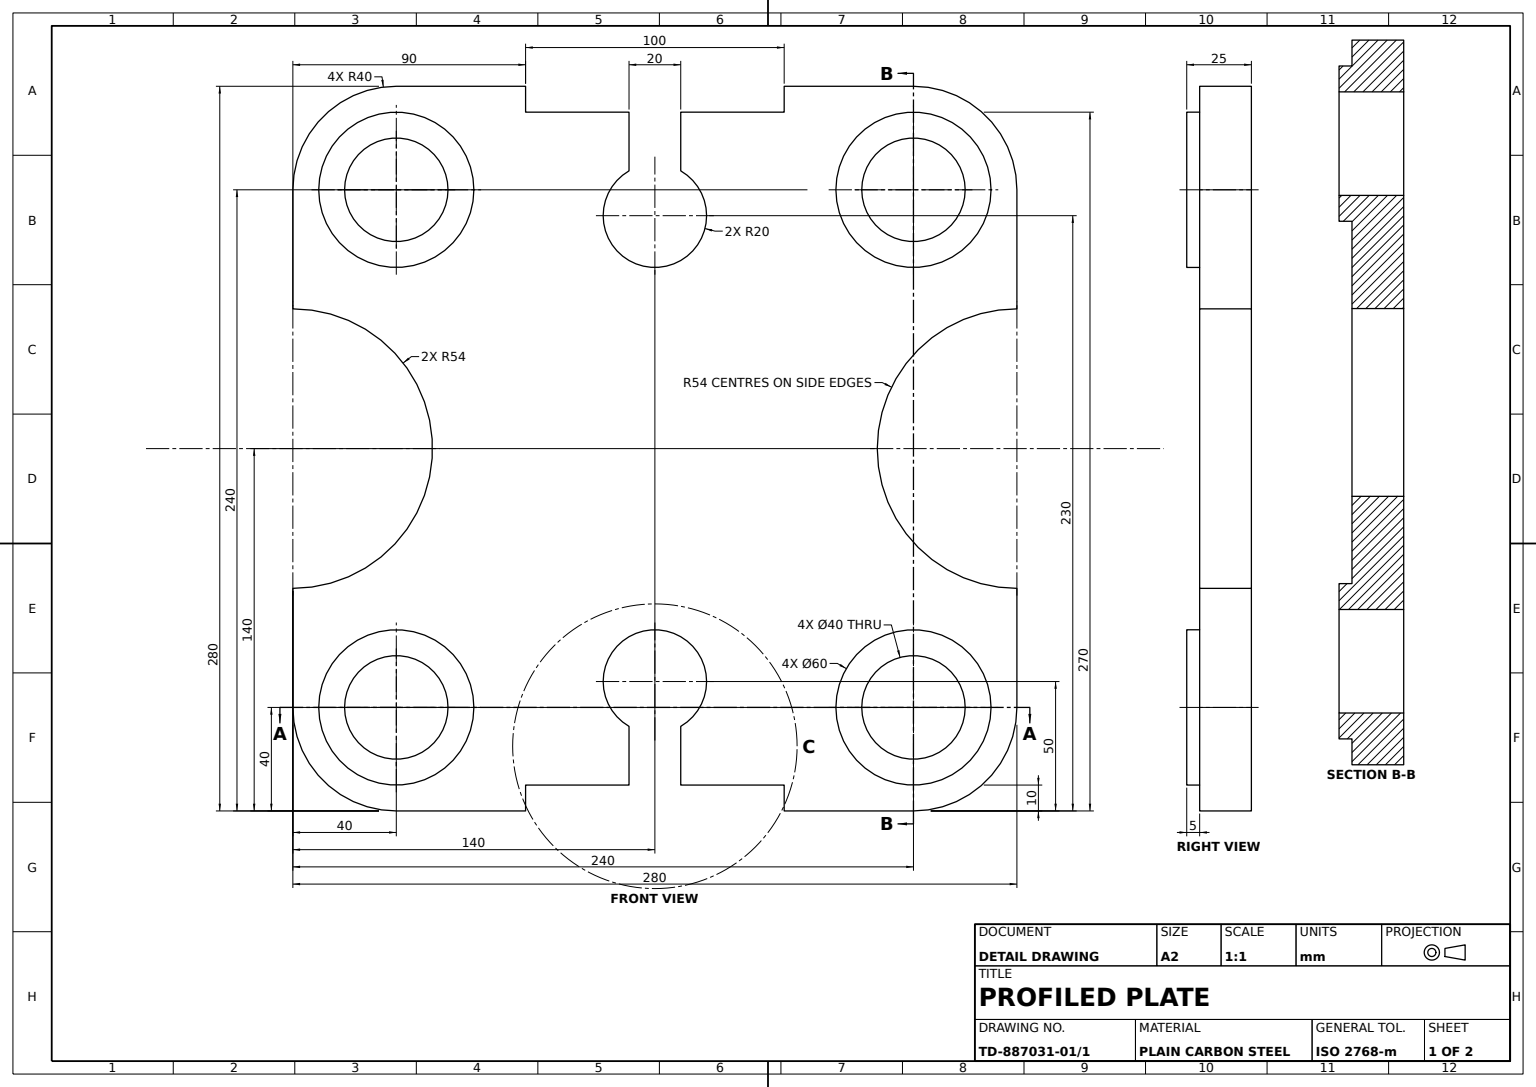
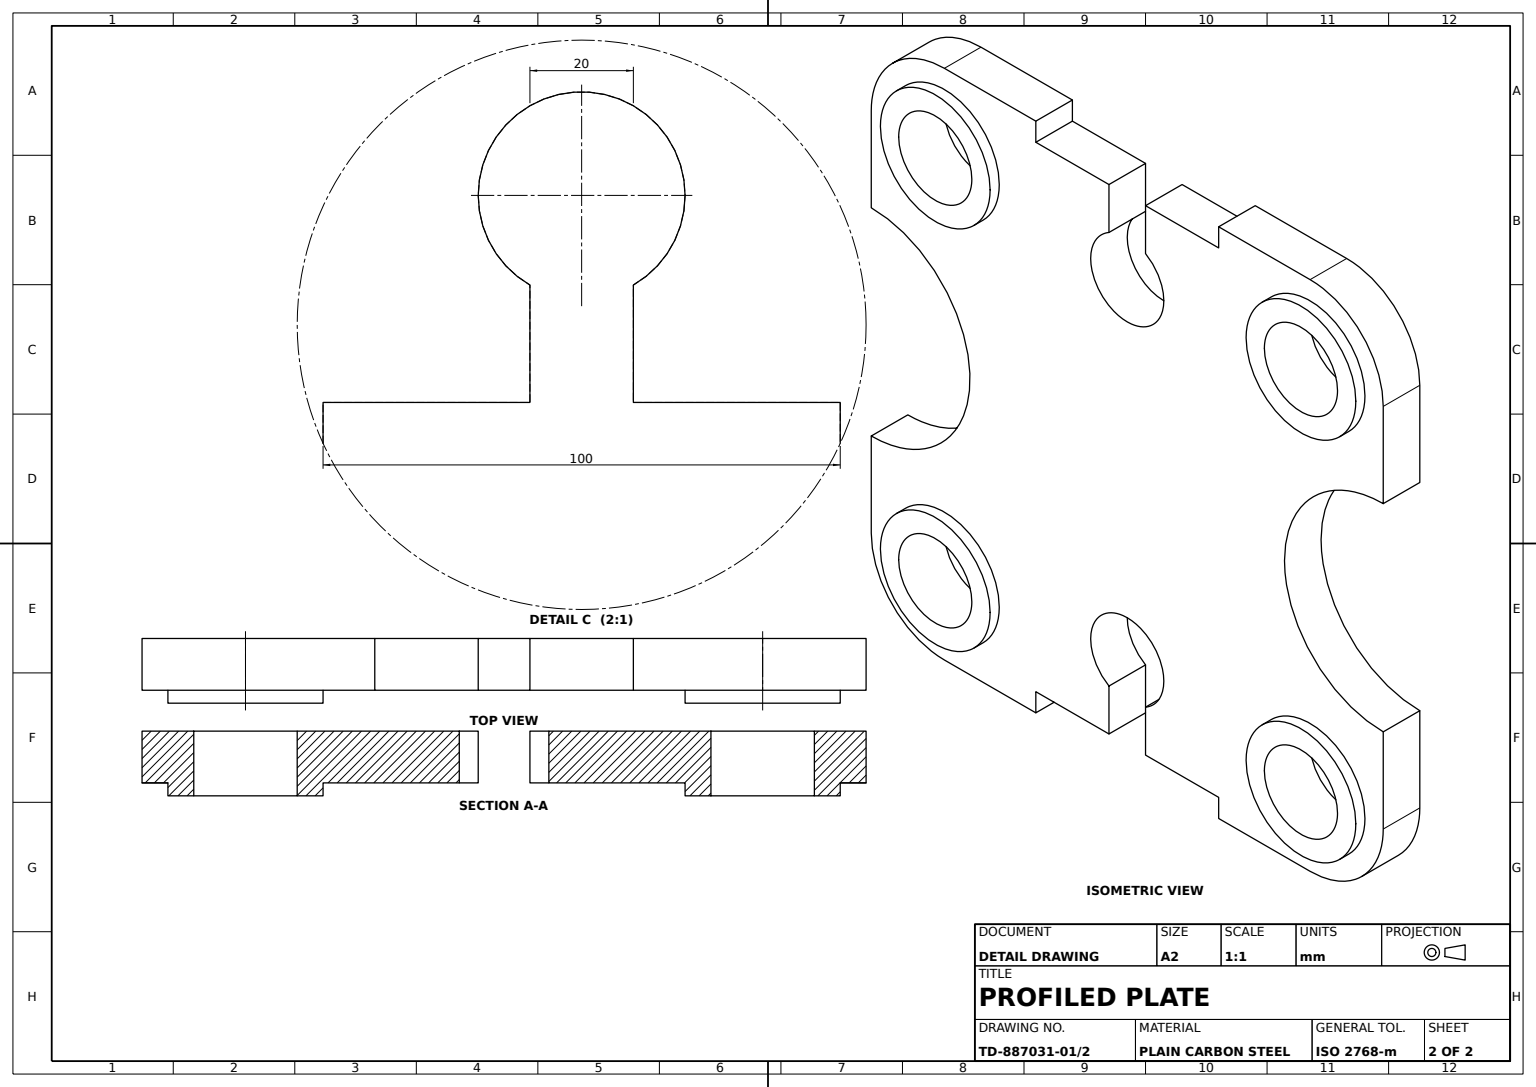
ISO-10303-21;
HEADER;
FILE_DESCRIPTION((''),'2;1');
FILE_NAME('','',(''),(''),'','','');
FILE_SCHEMA(('AUTOMOTIVE_DESIGN'));
ENDSEC;
DATA;
#1=APPLICATION_CONTEXT('');
#2=PRODUCT_CONTEXT('',#1,'mechanical');
#3=PRODUCT('','','',(#2));
#4=PRODUCT_DEFINITION_FORMATION('','',#3);
#5=PRODUCT_DEFINITION_CONTEXT('',#1,'design');
#6=PRODUCT_DEFINITION('','',#4,#5);
#7=PRODUCT_DEFINITION_SHAPE('','',#6);
#8=(LENGTH_UNIT()NAMED_UNIT(*)SI_UNIT(.MILLI.,.METRE.));
#9=(NAMED_UNIT(*)PLANE_ANGLE_UNIT()SI_UNIT($,.RADIAN.));
#10=(NAMED_UNIT(*)SI_UNIT($,.STERADIAN.)SOLID_ANGLE_UNIT());
#11=UNCERTAINTY_MEASURE_WITH_UNIT(LENGTH_MEASURE(1.E-05),#8,'distance_accuracy_value','');
#12=(GEOMETRIC_REPRESENTATION_CONTEXT(3)GLOBAL_UNCERTAINTY_ASSIGNED_CONTEXT((#11))GLOBAL_UNIT_ASSIGNED_CONTEXT((#8,#9,#10))REPRESENTATION_CONTEXT('',''));
#13=CARTESIAN_POINT('',(120.,230.,20.));
#14=VERTEX_POINT('',#13);
#15=CARTESIAN_POINT('',(120.,230.,0.));
#16=VERTEX_POINT('',#15);
#17=DIRECTION('',(0.,0.,-1.));
#18=VECTOR('',#17,1000.);
#19=LINE('',#13,#18);
#20=EDGE_CURVE('',#14,#16,#19,.T.);
#21=ORIENTED_EDGE('',*,*,#20,.T.);
#22=CARTESIAN_POINT('',(130.,247.320508,0.));
#23=VERTEX_POINT('',#22);
#24=CARTESIAN_POINT('',(140.,230.,0.));
#25=DIRECTION('',(1.,0.,0.));
#26=AXIS2_PLACEMENT_3D('',#24,#17,#25);
#27=CIRCLE('',#26,20.);
#28=EDGE_CURVE('',#16,#23,#27,.T.);
#29=ORIENTED_EDGE('',*,*,#28,.T.);
#30=CARTESIAN_POINT('',(130.,247.320508,20.));
#31=VERTEX_POINT('',#30);
#32=LINE('',#30,#18);
#33=EDGE_CURVE('',#31,#23,#32,.T.);
#34=ORIENTED_EDGE('',*,*,#33,.F.);
#35=CARTESIAN_POINT('',(140.,230.,20.));
#36=AXIS2_PLACEMENT_3D('',#35,#17,#25);
#37=CIRCLE('',#36,20.);
#38=EDGE_CURVE('',#14,#31,#37,.T.);
#39=ORIENTED_EDGE('',*,*,#38,.F.);
#40=EDGE_LOOP('',(#21,#29,#34,#39));
#41=FACE_OUTER_BOUND('',#40,.T.);
#42=DIRECTION('',(-1.,0.,0.));
#43=AXIS2_PLACEMENT_3D('',#35,#17,#42);
#44=CYLINDRICAL_SURFACE('',#43,20.);
#45=ADVANCED_FACE('',(#41),#44,.F.);
#46=CARTESIAN_POINT('',(240.,280.,20.));
#47=VERTEX_POINT('',#46);
#48=CARTESIAN_POINT('',(240.,280.,0.));
#49=VERTEX_POINT('',#48);
#50=LINE('',#46,#18);
#51=EDGE_CURVE('',#47,#49,#50,.T.);
#52=ORIENTED_EDGE('',*,*,#51,.T.);
#53=CARTESIAN_POINT('',(190.,280.,0.));
#54=VERTEX_POINT('',#53);
#55=VECTOR('',#42,1000.);
#56=LINE('',#48,#55);
#57=EDGE_CURVE('',#49,#54,#56,.T.);
#58=ORIENTED_EDGE('',*,*,#57,.T.);
#59=CARTESIAN_POINT('',(190.,280.,20.));
#60=VERTEX_POINT('',#59);
#61=LINE('',#59,#18);
#62=EDGE_CURVE('',#60,#54,#61,.T.);
#63=ORIENTED_EDGE('',*,*,#62,.F.);
#64=LINE('',#46,#55);
#65=EDGE_CURVE('',#47,#60,#64,.T.);
#66=ORIENTED_EDGE('',*,*,#65,.F.);
#67=EDGE_LOOP('',(#52,#58,#63,#66));
#68=FACE_OUTER_BOUND('',#67,.T.);
#69=DIRECTION('',(0.,-1.,0.));
#70=AXIS2_PLACEMENT_3D('',#46,#69,#25);
#71=PLANE('',#70);
#72=ADVANCED_FACE('',(#68),#71,.F.);
#73=CARTESIAN_POINT('',(90.,270.,20.));
#74=VERTEX_POINT('',#73);
#75=CARTESIAN_POINT('',(90.,270.,0.));
#76=VERTEX_POINT('',#75);
#77=LINE('',#73,#18);
#78=EDGE_CURVE('',#74,#76,#77,.T.);
#79=ORIENTED_EDGE('',*,*,#78,.T.);
#80=CARTESIAN_POINT('',(90.,280.,0.));
#81=VERTEX_POINT('',#80);
#82=DIRECTION('',(0.,1.,0.));
#83=VECTOR('',#82,1000.);
#84=LINE('',#75,#83);
#85=EDGE_CURVE('',#76,#81,#84,.T.);
#86=ORIENTED_EDGE('',*,*,#85,.T.);
#87=CARTESIAN_POINT('',(90.,280.,20.));
#88=VERTEX_POINT('',#87);
#89=LINE('',#87,#18);
#90=EDGE_CURVE('',#88,#81,#89,.T.);
#91=ORIENTED_EDGE('',*,*,#90,.F.);
#92=LINE('',#73,#83);
#93=EDGE_CURVE('',#74,#88,#92,.T.);
#94=ORIENTED_EDGE('',*,*,#93,.F.);
#95=EDGE_LOOP('',(#79,#86,#91,#94));
#96=FACE_OUTER_BOUND('',#95,.T.);
#97=DIRECTION('',(0.,0.,1.));
#98=AXIS2_PLACEMENT_3D('',#73,#42,#97);
#99=PLANE('',#98);
#100=ADVANCED_FACE('',(#96),#99,.F.);
#101=CARTESIAN_POINT('',(220.,240.,0.));
#102=VERTEX_POINT('',#101);
#103=CARTESIAN_POINT('',(260.,240.,0.));
#104=VERTEX_POINT('',#103);
#105=CARTESIAN_POINT('',(240.,240.,0.));
#106=AXIS2_PLACEMENT_3D('',#105,#97,#25);
#107=CIRCLE('',#106,20.);
#108=EDGE_CURVE('',#102,#104,#107,.T.);
#109=ORIENTED_EDGE('',*,*,#108,.T.);
#110=EDGE_CURVE('',#104,#102,#107,.T.);
#111=ORIENTED_EDGE('',*,*,#110,.T.);
#112=EDGE_LOOP('',(#109,#111));
#113=FACE_BOUND('',#112,.T.);
#114=CARTESIAN_POINT('',(20.,240.,0.));
#115=VERTEX_POINT('',#114);
#116=CARTESIAN_POINT('',(60.,240.,0.));
#117=VERTEX_POINT('',#116);
#118=CARTESIAN_POINT('',(40.,240.,0.));
#119=AXIS2_PLACEMENT_3D('',#118,#97,#25);
#120=CIRCLE('',#119,20.);
#121=EDGE_CURVE('',#115,#117,#120,.T.);
#122=ORIENTED_EDGE('',*,*,#121,.T.);
#123=EDGE_CURVE('',#117,#115,#120,.T.);
#124=ORIENTED_EDGE('',*,*,#123,.T.);
#125=EDGE_LOOP('',(#122,#124));
#126=FACE_BOUND('',#125,.T.);
#127=ORIENTED_EDGE('',*,*,#28,.F.);
#128=CARTESIAN_POINT('',(160.,230.,0.));
#129=VERTEX_POINT('',#128);
#130=EDGE_CURVE('',#129,#16,#27,.T.);
#131=ORIENTED_EDGE('',*,*,#130,.F.);
#132=CARTESIAN_POINT('',(150.,247.320508,0.));
#133=VERTEX_POINT('',#132);
#134=EDGE_CURVE('',#133,#129,#27,.T.);
#135=ORIENTED_EDGE('',*,*,#134,.F.);
#136=CARTESIAN_POINT('',(150.,270.,0.));
#137=VERTEX_POINT('',#136);
#138=VECTOR('',#69,1000.);
#139=LINE('',#136,#138);
#140=EDGE_CURVE('',#137,#133,#139,.T.);
#141=ORIENTED_EDGE('',*,*,#140,.F.);
#142=CARTESIAN_POINT('',(190.,270.,0.));
#143=VERTEX_POINT('',#142);
#144=LINE('',#142,#55);
#145=EDGE_CURVE('',#143,#137,#144,.T.);
#146=ORIENTED_EDGE('',*,*,#145,.F.);
#147=LINE('',#53,#138);
#148=EDGE_CURVE('',#54,#143,#147,.T.);
#149=ORIENTED_EDGE('',*,*,#148,.F.);
#150=ORIENTED_EDGE('',*,*,#57,.F.);
#151=CARTESIAN_POINT('',(280.,240.,0.));
#152=VERTEX_POINT('',#151);
#153=AXIS2_PLACEMENT_3D('',#105,#97,#42);
#154=CIRCLE('',#153,40.);
#155=EDGE_CURVE('',#152,#49,#154,.T.);
#156=ORIENTED_EDGE('',*,*,#155,.F.);
#157=CARTESIAN_POINT('',(280.,194.,0.));
#158=VERTEX_POINT('',#157);
#159=LINE('',#157,#83);
#160=EDGE_CURVE('',#158,#152,#159,.T.);
#161=ORIENTED_EDGE('',*,*,#160,.F.);
#162=CARTESIAN_POINT('',(226.,140.,0.));
#163=VERTEX_POINT('',#162);
#164=CARTESIAN_POINT('',(280.,140.,0.));
#165=AXIS2_PLACEMENT_3D('',#164,#17,#25);
#166=CIRCLE('',#165,54.);
#167=EDGE_CURVE('',#163,#158,#166,.T.);
#168=ORIENTED_EDGE('',*,*,#167,.F.);
#169=CARTESIAN_POINT('',(280.,86.,0.));
#170=VERTEX_POINT('',#169);
#171=EDGE_CURVE('',#170,#163,#166,.T.);
#172=ORIENTED_EDGE('',*,*,#171,.F.);
#173=CARTESIAN_POINT('',(280.,40.,0.));
#174=VERTEX_POINT('',#173);
#175=LINE('',#173,#83);
#176=EDGE_CURVE('',#174,#170,#175,.T.);
#177=ORIENTED_EDGE('',*,*,#176,.F.);
#178=CARTESIAN_POINT('',(240.,0.,0.));
#179=VERTEX_POINT('',#178);
#180=CARTESIAN_POINT('',(240.,40.,0.));
#181=AXIS2_PLACEMENT_3D('',#180,#97,#42);
#182=CIRCLE('',#181,40.);
#183=EDGE_CURVE('',#179,#174,#182,.T.);
#184=ORIENTED_EDGE('',*,*,#183,.F.);
#185=CARTESIAN_POINT('',(190.,0.,0.));
#186=VERTEX_POINT('',#185);
#187=VECTOR('',#25,1000.);
#188=LINE('',#185,#187);
#189=EDGE_CURVE('',#186,#179,#188,.T.);
#190=ORIENTED_EDGE('',*,*,#189,.F.);
#191=CARTESIAN_POINT('',(190.,10.,0.));
#192=VERTEX_POINT('',#191);
#193=LINE('',#191,#138);
#194=EDGE_CURVE('',#192,#186,#193,.T.);
#195=ORIENTED_EDGE('',*,*,#194,.F.);
#196=CARTESIAN_POINT('',(150.,10.,0.));
#197=VERTEX_POINT('',#196);
#198=LINE('',#196,#187);
#199=EDGE_CURVE('',#197,#192,#198,.T.);
#200=ORIENTED_EDGE('',*,*,#199,.F.);
#201=CARTESIAN_POINT('',(150.,32.679492,0.));
#202=VERTEX_POINT('',#201);
#203=LINE('',#196,#138);
#204=EDGE_CURVE('',#202,#197,#203,.T.);
#205=ORIENTED_EDGE('',*,*,#204,.F.);
#206=CARTESIAN_POINT('',(160.,50.,0.));
#207=VERTEX_POINT('',#206);
#208=CARTESIAN_POINT('',(140.,50.,0.));
#209=AXIS2_PLACEMENT_3D('',#208,#17,#25);
#210=CIRCLE('',#209,20.);
#211=EDGE_CURVE('',#207,#202,#210,.T.);
#212=ORIENTED_EDGE('',*,*,#211,.F.);
#213=CARTESIAN_POINT('',(120.,50.,0.));
#214=VERTEX_POINT('',#213);
#215=EDGE_CURVE('',#214,#207,#210,.T.);
#216=ORIENTED_EDGE('',*,*,#215,.F.);
#217=CARTESIAN_POINT('',(130.,32.679492,0.));
#218=VERTEX_POINT('',#217);
#219=EDGE_CURVE('',#218,#214,#210,.T.);
#220=ORIENTED_EDGE('',*,*,#219,.F.);
#221=CARTESIAN_POINT('',(130.,10.,0.));
#222=VERTEX_POINT('',#221);
#223=LINE('',#221,#83);
#224=EDGE_CURVE('',#222,#218,#223,.T.);
#225=ORIENTED_EDGE('',*,*,#224,.F.);
#226=CARTESIAN_POINT('',(90.,10.,0.));
#227=VERTEX_POINT('',#226);
#228=LINE('',#226,#187);
#229=EDGE_CURVE('',#227,#222,#228,.T.);
#230=ORIENTED_EDGE('',*,*,#229,.F.);
#231=CARTESIAN_POINT('',(90.,0.,0.));
#232=VERTEX_POINT('',#231);
#233=LINE('',#231,#83);
#234=EDGE_CURVE('',#232,#227,#233,.T.);
#235=ORIENTED_EDGE('',*,*,#234,.F.);
#236=CARTESIAN_POINT('',(40.,0.,0.));
#237=VERTEX_POINT('',#236);
#238=LINE('',#236,#187);
#239=EDGE_CURVE('',#237,#232,#238,.T.);
#240=ORIENTED_EDGE('',*,*,#239,.F.);
#241=CARTESIAN_POINT('',(0.,40.,0.));
#242=VERTEX_POINT('',#241);
#243=CARTESIAN_POINT('',(40.,40.,0.));
#244=AXIS2_PLACEMENT_3D('',#243,#97,#42);
#245=CIRCLE('',#244,40.);
#246=EDGE_CURVE('',#242,#237,#245,.T.);
#247=ORIENTED_EDGE('',*,*,#246,.F.);
#248=CARTESIAN_POINT('',(0.,86.,0.));
#249=VERTEX_POINT('',#248);
#250=LINE('',#248,#138);
#251=EDGE_CURVE('',#249,#242,#250,.T.);
#252=ORIENTED_EDGE('',*,*,#251,.F.);
#253=CARTESIAN_POINT('',(0.,194.,0.));
#254=VERTEX_POINT('',#253);
#255=CARTESIAN_POINT('',(0.,140.,0.));
#256=AXIS2_PLACEMENT_3D('',#255,#17,#25);
#257=CIRCLE('',#256,54.);
#258=EDGE_CURVE('',#254,#249,#257,.T.);
#259=ORIENTED_EDGE('',*,*,#258,.F.);
#260=CARTESIAN_POINT('',(0.,240.,0.));
#261=VERTEX_POINT('',#260);
#262=LINE('',#260,#138);
#263=EDGE_CURVE('',#261,#254,#262,.T.);
#264=ORIENTED_EDGE('',*,*,#263,.F.);
#265=CARTESIAN_POINT('',(40.,280.,0.));
#266=VERTEX_POINT('',#265);
#267=AXIS2_PLACEMENT_3D('',#118,#97,#42);
#268=CIRCLE('',#267,40.);
#269=EDGE_CURVE('',#266,#261,#268,.T.);
#270=ORIENTED_EDGE('',*,*,#269,.F.);
#271=LINE('',#80,#55);
#272=EDGE_CURVE('',#81,#266,#271,.T.);
#273=ORIENTED_EDGE('',*,*,#272,.F.);
#274=ORIENTED_EDGE('',*,*,#85,.F.);
#275=CARTESIAN_POINT('',(130.,270.,0.));
#276=VERTEX_POINT('',#275);
#277=LINE('',#275,#55);
#278=EDGE_CURVE('',#276,#76,#277,.T.);
#279=ORIENTED_EDGE('',*,*,#278,.F.);
#280=LINE('',#275,#83);
#281=EDGE_CURVE('',#23,#276,#280,.T.);
#282=ORIENTED_EDGE('',*,*,#281,.F.);
#283=EDGE_LOOP('',(#127,#131,#135,#141,#146,#149,#150,#156,#161,#168,#172,#177,#184,#190,#195,#200,#205,#212,#216,#220,#225,#230,#235,#240,#247,#252,#259,#264,#270,#273,#274,#279,#282));
#284=FACE_OUTER_BOUND('',#283,.T.);
#285=CARTESIAN_POINT('',(220.,40.,0.));
#286=VERTEX_POINT('',#285);
#287=CARTESIAN_POINT('',(260.,40.,0.));
#288=VERTEX_POINT('',#287);
#289=AXIS2_PLACEMENT_3D('',#180,#97,#25);
#290=CIRCLE('',#289,20.);
#291=EDGE_CURVE('',#286,#288,#290,.T.);
#292=ORIENTED_EDGE('',*,*,#291,.T.);
#293=EDGE_CURVE('',#288,#286,#290,.T.);
#294=ORIENTED_EDGE('',*,*,#293,.T.);
#295=EDGE_LOOP('',(#292,#294));
#296=FACE_BOUND('',#295,.T.);
#297=CARTESIAN_POINT('',(20.,40.,0.));
#298=VERTEX_POINT('',#297);
#299=CARTESIAN_POINT('',(60.,40.,0.));
#300=VERTEX_POINT('',#299);
#301=AXIS2_PLACEMENT_3D('',#243,#97,#25);
#302=CIRCLE('',#301,20.);
#303=EDGE_CURVE('',#298,#300,#302,.T.);
#304=ORIENTED_EDGE('',*,*,#303,.T.);
#305=EDGE_CURVE('',#300,#298,#302,.T.);
#306=ORIENTED_EDGE('',*,*,#305,.T.);
#307=EDGE_LOOP('',(#304,#306));
#308=FACE_BOUND('',#307,.T.);
#309=AXIS2_PLACEMENT_3D('',#208,#97,#25);
#310=PLANE('',#309);
#311=ADVANCED_FACE('',(#113,#126,#284,#296,#308),#310,.F.);
#312=ORIENTED_EDGE('',*,*,#140,.T.);
#313=CARTESIAN_POINT('',(150.,247.320508,20.));
#314=VERTEX_POINT('',#313);
#315=LINE('',#313,#18);
#316=EDGE_CURVE('',#314,#133,#315,.T.);
#317=ORIENTED_EDGE('',*,*,#316,.F.);
#318=CARTESIAN_POINT('',(150.,270.,20.));
#319=VERTEX_POINT('',#318);
#320=LINE('',#318,#138);
#321=EDGE_CURVE('',#319,#314,#320,.T.);
#322=ORIENTED_EDGE('',*,*,#321,.F.);
#323=LINE('',#318,#18);
#324=EDGE_CURVE('',#319,#137,#323,.T.);
#325=ORIENTED_EDGE('',*,*,#324,.T.);
#326=EDGE_LOOP('',(#312,#317,#322,#325));
#327=FACE_OUTER_BOUND('',#326,.T.);
#328=AXIS2_PLACEMENT_3D('',#318,#25,#17);
#329=PLANE('',#328);
#330=ADVANCED_FACE('',(#327),#329,.F.);
#331=CARTESIAN_POINT('',(40.,280.,20.));
#332=VERTEX_POINT('',#331);
#333=LINE('',#87,#55);
#334=EDGE_CURVE('',#88,#332,#333,.T.);
#335=ORIENTED_EDGE('',*,*,#334,.F.);
#336=ORIENTED_EDGE('',*,*,#90,.T.);
#337=ORIENTED_EDGE('',*,*,#272,.T.);
#338=LINE('',#331,#18);
#339=EDGE_CURVE('',#332,#266,#338,.T.);
#340=ORIENTED_EDGE('',*,*,#339,.F.);
#341=EDGE_LOOP('',(#335,#336,#337,#340));
#342=FACE_OUTER_BOUND('',#341,.T.);
#343=AXIS2_PLACEMENT_3D('',#87,#69,#17);
#344=PLANE('',#343);
#345=ADVANCED_FACE('',(#342),#344,.F.);
#346=CARTESIAN_POINT('',(190.,0.,20.));
#347=VERTEX_POINT('',#346);
#348=CARTESIAN_POINT('',(240.,0.,20.));
#349=VERTEX_POINT('',#348);
#350=LINE('',#346,#187);
#351=EDGE_CURVE('',#347,#349,#350,.T.);
#352=ORIENTED_EDGE('',*,*,#351,.F.);
#353=LINE('',#346,#18);
#354=EDGE_CURVE('',#347,#186,#353,.T.);
#355=ORIENTED_EDGE('',*,*,#354,.T.);
#356=ORIENTED_EDGE('',*,*,#189,.T.);
#357=LINE('',#348,#18);
#358=EDGE_CURVE('',#349,#179,#357,.T.);
#359=ORIENTED_EDGE('',*,*,#358,.F.);
#360=EDGE_LOOP('',(#352,#355,#356,#359));
#361=FACE_OUTER_BOUND('',#360,.T.);
#362=AXIS2_PLACEMENT_3D('',#346,#82,#42);
#363=PLANE('',#362);
#364=ADVANCED_FACE('',(#361),#363,.F.);
#365=ORIENTED_EDGE('',*,*,#219,.T.);
#366=CARTESIAN_POINT('',(120.,50.,20.));
#367=VERTEX_POINT('',#366);
#368=LINE('',#366,#18);
#369=EDGE_CURVE('',#367,#214,#368,.T.);
#370=ORIENTED_EDGE('',*,*,#369,.F.);
#371=CARTESIAN_POINT('',(130.,32.679492,20.));
#372=VERTEX_POINT('',#371);
#373=CARTESIAN_POINT('',(140.,50.,20.));
#374=AXIS2_PLACEMENT_3D('',#373,#17,#25);
#375=CIRCLE('',#374,20.);
#376=EDGE_CURVE('',#372,#367,#375,.T.);
#377=ORIENTED_EDGE('',*,*,#376,.F.);
#378=LINE('',#371,#18);
#379=EDGE_CURVE('',#372,#218,#378,.T.);
#380=ORIENTED_EDGE('',*,*,#379,.T.);
#381=EDGE_LOOP('',(#365,#370,#377,#380));
#382=FACE_OUTER_BOUND('',#381,.T.);
#383=AXIS2_PLACEMENT_3D('',#373,#17,#42);
#384=CYLINDRICAL_SURFACE('',#383,20.);
#385=ADVANCED_FACE('',(#382),#384,.F.);
#386=ORIENTED_EDGE('',*,*,#160,.T.);
#387=CARTESIAN_POINT('',(280.,240.,20.));
#388=VERTEX_POINT('',#387);
#389=LINE('',#387,#18);
#390=EDGE_CURVE('',#388,#152,#389,.T.);
#391=ORIENTED_EDGE('',*,*,#390,.F.);
#392=CARTESIAN_POINT('',(280.,194.,20.));
#393=VERTEX_POINT('',#392);
#394=LINE('',#392,#83);
#395=EDGE_CURVE('',#393,#388,#394,.T.);
#396=ORIENTED_EDGE('',*,*,#395,.F.);
#397=LINE('',#392,#18);
#398=EDGE_CURVE('',#393,#158,#397,.T.);
#399=ORIENTED_EDGE('',*,*,#398,.T.);
#400=EDGE_LOOP('',(#386,#391,#396,#399));
#401=FACE_OUTER_BOUND('',#400,.T.);
#402=AXIS2_PLACEMENT_3D('',#392,#42,#97);
#403=PLANE('',#402);
#404=ADVANCED_FACE('',(#401),#403,.F.);
#405=CARTESIAN_POINT('',(10.,40.,25.));
#406=VERTEX_POINT('',#405);
#407=CARTESIAN_POINT('',(70.,40.,25.));
#408=VERTEX_POINT('',#407);
#409=CARTESIAN_POINT('',(40.,40.,25.));
#410=AXIS2_PLACEMENT_3D('',#409,#97,#25);
#411=CIRCLE('',#410,30.);
#412=EDGE_CURVE('',#406,#408,#411,.T.);
#413=ORIENTED_EDGE('',*,*,#412,.T.);
#414=EDGE_CURVE('',#408,#406,#411,.T.);
#415=ORIENTED_EDGE('',*,*,#414,.T.);
#416=EDGE_LOOP('',(#413,#415));
#417=FACE_OUTER_BOUND('',#416,.T.);
#418=CARTESIAN_POINT('',(20.,40.,25.));
#419=VERTEX_POINT('',#418);
#420=CARTESIAN_POINT('',(60.,40.,25.));
#421=VERTEX_POINT('',#420);
#422=CIRCLE('',#410,20.);
#423=EDGE_CURVE('',#419,#421,#422,.T.);
#424=ORIENTED_EDGE('',*,*,#423,.F.);
#425=EDGE_CURVE('',#421,#419,#422,.T.);
#426=ORIENTED_EDGE('',*,*,#425,.F.);
#427=EDGE_LOOP('',(#424,#426));
#428=FACE_BOUND('',#427,.T.);
#429=PLANE('',#410);
#430=ADVANCED_FACE('',(#417,#428),#429,.T.);
#431=CARTESIAN_POINT('',(10.,240.,25.));
#432=VERTEX_POINT('',#431);
#433=CARTESIAN_POINT('',(10.,240.,20.));
#434=VERTEX_POINT('',#433);
#435=LINE('',#431,#18);
#436=EDGE_CURVE('',#432,#434,#435,.T.);
#437=ORIENTED_EDGE('',*,*,#436,.T.);
#438=CARTESIAN_POINT('',(70.,240.,20.));
#439=VERTEX_POINT('',#438);
#440=CARTESIAN_POINT('',(40.,240.,20.));
#441=AXIS2_PLACEMENT_3D('',#440,#97,#25);
#442=CIRCLE('',#441,30.);
#443=EDGE_CURVE('',#434,#439,#442,.T.);
#444=ORIENTED_EDGE('',*,*,#443,.T.);
#445=CARTESIAN_POINT('',(70.,240.,25.));
#446=VERTEX_POINT('',#445);
#447=LINE('',#445,#18);
#448=EDGE_CURVE('',#446,#439,#447,.T.);
#449=ORIENTED_EDGE('',*,*,#448,.F.);
#450=CARTESIAN_POINT('',(40.,240.,25.));
#451=AXIS2_PLACEMENT_3D('',#450,#97,#25);
#452=CIRCLE('',#451,30.);
#453=EDGE_CURVE('',#432,#446,#452,.T.);
#454=ORIENTED_EDGE('',*,*,#453,.F.);
#455=EDGE_LOOP('',(#437,#444,#449,#454));
#456=FACE_OUTER_BOUND('',#455,.T.);
#457=AXIS2_PLACEMENT_3D('',#450,#17,#42);
#458=CYLINDRICAL_SURFACE('',#457,30.);
#459=ADVANCED_FACE('',(#456),#458,.T.);
#460=CARTESIAN_POINT('',(280.,86.,20.));
#461=VERTEX_POINT('',#460);
#462=LINE('',#460,#18);
#463=EDGE_CURVE('',#461,#170,#462,.T.);
#464=ORIENTED_EDGE('',*,*,#463,.T.);
#465=ORIENTED_EDGE('',*,*,#171,.T.);
#466=CARTESIAN_POINT('',(226.,140.,20.));
#467=VERTEX_POINT('',#466);
#468=LINE('',#466,#18);
#469=EDGE_CURVE('',#467,#163,#468,.T.);
#470=ORIENTED_EDGE('',*,*,#469,.F.);
#471=CARTESIAN_POINT('',(280.,140.,20.));
#472=AXIS2_PLACEMENT_3D('',#471,#17,#25);
#473=CIRCLE('',#472,54.);
#474=EDGE_CURVE('',#461,#467,#473,.T.);
#475=ORIENTED_EDGE('',*,*,#474,.F.);
#476=EDGE_LOOP('',(#464,#465,#470,#475));
#477=FACE_OUTER_BOUND('',#476,.T.);
#478=AXIS2_PLACEMENT_3D('',#471,#17,#42);
#479=CYLINDRICAL_SURFACE('',#478,54.);
#480=ADVANCED_FACE('',(#477),#479,.F.);
#481=ORIENTED_EDGE('',*,*,#167,.T.);
#482=ORIENTED_EDGE('',*,*,#398,.F.);
#483=EDGE_CURVE('',#467,#393,#473,.T.);
#484=ORIENTED_EDGE('',*,*,#483,.F.);
#485=ORIENTED_EDGE('',*,*,#469,.T.);
#486=EDGE_LOOP('',(#481,#482,#484,#485));
#487=FACE_OUTER_BOUND('',#486,.T.);
#488=ADVANCED_FACE('',(#487),#479,.F.);
#489=CARTESIAN_POINT('',(220.,40.,25.));
#490=VERTEX_POINT('',#489);
#491=CARTESIAN_POINT('',(260.,40.,25.));
#492=VERTEX_POINT('',#491);
#493=CARTESIAN_POINT('',(240.,40.,25.));
#494=AXIS2_PLACEMENT_3D('',#493,#97,#25);
#495=CIRCLE('',#494,20.);
#496=EDGE_CURVE('',#490,#492,#495,.T.);
#497=ORIENTED_EDGE('',*,*,#496,.F.);
#498=EDGE_CURVE('',#492,#490,#495,.T.);
#499=ORIENTED_EDGE('',*,*,#498,.F.);
#500=EDGE_LOOP('',(#497,#499));
#501=FACE_BOUND('',#500,.T.);
#502=CARTESIAN_POINT('',(270.,40.,25.));
#503=VERTEX_POINT('',#502);
#504=CARTESIAN_POINT('',(210.,40.,25.));
#505=VERTEX_POINT('',#504);
#506=CIRCLE('',#494,30.);
#507=EDGE_CURVE('',#503,#505,#506,.T.);
#508=ORIENTED_EDGE('',*,*,#507,.T.);
#509=EDGE_CURVE('',#505,#503,#506,.T.);
#510=ORIENTED_EDGE('',*,*,#509,.T.);
#511=EDGE_LOOP('',(#508,#510));
#512=FACE_OUTER_BOUND('',#511,.T.);
#513=PLANE('',#494);
#514=ADVANCED_FACE('',(#501,#512),#513,.T.);
#515=ORIENTED_EDGE('',*,*,#269,.T.);
#516=CARTESIAN_POINT('',(0.,240.,20.));
#517=VERTEX_POINT('',#516);
#518=LINE('',#516,#18);
#519=EDGE_CURVE('',#517,#261,#518,.T.);
#520=ORIENTED_EDGE('',*,*,#519,.F.);
#521=AXIS2_PLACEMENT_3D('',#440,#97,#42);
#522=CIRCLE('',#521,40.);
#523=EDGE_CURVE('',#332,#517,#522,.T.);
#524=ORIENTED_EDGE('',*,*,#523,.F.);
#525=ORIENTED_EDGE('',*,*,#339,.T.);
#526=EDGE_LOOP('',(#515,#520,#524,#525));
#527=FACE_OUTER_BOUND('',#526,.T.);
#528=AXIS2_PLACEMENT_3D('',#440,#17,#42);
#529=CYLINDRICAL_SURFACE('',#528,40.);
#530=ADVANCED_FACE('',(#527),#529,.T.);
#531=CARTESIAN_POINT('',(210.,240.,25.));
#532=VERTEX_POINT('',#531);
#533=CARTESIAN_POINT('',(270.,240.,25.));
#534=VERTEX_POINT('',#533);
#535=CARTESIAN_POINT('',(240.,240.,25.));
#536=AXIS2_PLACEMENT_3D('',#535,#97,#25);
#537=CIRCLE('',#536,30.);
#538=EDGE_CURVE('',#532,#534,#537,.T.);
#539=ORIENTED_EDGE('',*,*,#538,.T.);
#540=EDGE_CURVE('',#534,#532,#537,.T.);
#541=ORIENTED_EDGE('',*,*,#540,.T.);
#542=EDGE_LOOP('',(#539,#541));
#543=FACE_OUTER_BOUND('',#542,.T.);
#544=CARTESIAN_POINT('',(220.,240.,25.));
#545=VERTEX_POINT('',#544);
#546=CARTESIAN_POINT('',(260.,240.,25.));
#547=VERTEX_POINT('',#546);
#548=CIRCLE('',#536,20.);
#549=EDGE_CURVE('',#545,#547,#548,.T.);
#550=ORIENTED_EDGE('',*,*,#549,.F.);
#551=EDGE_CURVE('',#547,#545,#548,.T.);
#552=ORIENTED_EDGE('',*,*,#551,.F.);
#553=EDGE_LOOP('',(#550,#552));
#554=FACE_BOUND('',#553,.T.);
#555=PLANE('',#536);
#556=ADVANCED_FACE('',(#543,#554),#555,.T.);
#557=CARTESIAN_POINT('',(270.,240.,20.));
#558=VERTEX_POINT('',#557);
#559=CARTESIAN_POINT('',(210.,240.,20.));
#560=VERTEX_POINT('',#559);
#561=CARTESIAN_POINT('',(240.,240.,20.));
#562=AXIS2_PLACEMENT_3D('',#561,#97,#25);
#563=CIRCLE('',#562,30.);
#564=EDGE_CURVE('',#558,#560,#563,.T.);
#565=ORIENTED_EDGE('',*,*,#564,.T.);
#566=LINE('',#531,#18);
#567=EDGE_CURVE('',#532,#560,#566,.T.);
#568=ORIENTED_EDGE('',*,*,#567,.F.);
#569=ORIENTED_EDGE('',*,*,#540,.F.);
#570=LINE('',#533,#18);
#571=EDGE_CURVE('',#534,#558,#570,.T.);
#572=ORIENTED_EDGE('',*,*,#571,.T.);
#573=EDGE_LOOP('',(#565,#568,#569,#572));
#574=FACE_OUTER_BOUND('',#573,.T.);
#575=AXIS2_PLACEMENT_3D('',#535,#17,#42);
#576=CYLINDRICAL_SURFACE('',#575,30.);
#577=ADVANCED_FACE('',(#574),#576,.T.);
#578=CARTESIAN_POINT('',(0.,86.,20.));
#579=VERTEX_POINT('',#578);
#580=LINE('',#578,#18);
#581=EDGE_CURVE('',#579,#249,#580,.T.);
#582=ORIENTED_EDGE('',*,*,#581,.T.);
#583=ORIENTED_EDGE('',*,*,#251,.T.);
#584=CARTESIAN_POINT('',(0.,40.,20.));
#585=VERTEX_POINT('',#584);
#586=LINE('',#584,#18);
#587=EDGE_CURVE('',#585,#242,#586,.T.);
#588=ORIENTED_EDGE('',*,*,#587,.F.);
#589=LINE('',#578,#138);
#590=EDGE_CURVE('',#579,#585,#589,.T.);
#591=ORIENTED_EDGE('',*,*,#590,.F.);
#592=EDGE_LOOP('',(#582,#583,#588,#591));
#593=FACE_OUTER_BOUND('',#592,.T.);
#594=AXIS2_PLACEMENT_3D('',#578,#25,#17);
#595=PLANE('',#594);
#596=ADVANCED_FACE('',(#593),#595,.F.);
#597=CARTESIAN_POINT('',(130.,270.,20.));
#598=VERTEX_POINT('',#597);
#599=LINE('',#597,#18);
#600=EDGE_CURVE('',#598,#276,#599,.T.);
#601=ORIENTED_EDGE('',*,*,#600,.F.);
#602=LINE('',#597,#83);
#603=EDGE_CURVE('',#31,#598,#602,.T.);
#604=ORIENTED_EDGE('',*,*,#603,.F.);
#605=ORIENTED_EDGE('',*,*,#33,.T.);
#606=ORIENTED_EDGE('',*,*,#281,.T.);
#607=EDGE_LOOP('',(#601,#604,#605,#606));
#608=FACE_OUTER_BOUND('',#607,.T.);
#609=AXIS2_PLACEMENT_3D('',#597,#42,#97);
#610=PLANE('',#609);
#611=ADVANCED_FACE('',(#608),#610,.F.);
#612=ORIENTED_EDGE('',*,*,#305,.F.);
#613=LINE('',#420,#18);
#614=EDGE_CURVE('',#421,#300,#613,.T.);
#615=ORIENTED_EDGE('',*,*,#614,.F.);
#616=ORIENTED_EDGE('',*,*,#425,.T.);
#617=LINE('',#418,#18);
#618=EDGE_CURVE('',#419,#298,#617,.T.);
#619=ORIENTED_EDGE('',*,*,#618,.T.);
#620=EDGE_LOOP('',(#612,#615,#616,#619));
#621=FACE_OUTER_BOUND('',#620,.T.);
#622=AXIS2_PLACEMENT_3D('',#409,#17,#42);
#623=CYLINDRICAL_SURFACE('',#622,20.);
#624=ADVANCED_FACE('',(#621),#623,.F.);
#625=CARTESIAN_POINT('',(60.,240.,25.));
#626=VERTEX_POINT('',#625);
#627=CARTESIAN_POINT('',(20.,240.,25.));
#628=VERTEX_POINT('',#627);
#629=CIRCLE('',#451,20.);
#630=EDGE_CURVE('',#626,#628,#629,.T.);
#631=ORIENTED_EDGE('',*,*,#630,.T.);
#632=LINE('',#627,#18);
#633=EDGE_CURVE('',#628,#115,#632,.T.);
#634=ORIENTED_EDGE('',*,*,#633,.T.);
#635=ORIENTED_EDGE('',*,*,#123,.F.);
#636=LINE('',#625,#18);
#637=EDGE_CURVE('',#626,#117,#636,.T.);
#638=ORIENTED_EDGE('',*,*,#637,.F.);
#639=EDGE_LOOP('',(#631,#634,#635,#638));
#640=FACE_OUTER_BOUND('',#639,.T.);
#641=CYLINDRICAL_SURFACE('',#457,20.);
#642=ADVANCED_FACE('',(#640),#641,.F.);
#643=CARTESIAN_POINT('',(70.,40.,20.));
#644=VERTEX_POINT('',#643);
#645=LINE('',#407,#18);
#646=EDGE_CURVE('',#408,#644,#645,.T.);
#647=ORIENTED_EDGE('',*,*,#646,.T.);
#648=CARTESIAN_POINT('',(10.,40.,20.));
#649=VERTEX_POINT('',#648);
#650=CARTESIAN_POINT('',(40.,40.,20.));
#651=AXIS2_PLACEMENT_3D('',#650,#97,#25);
#652=CIRCLE('',#651,30.);
#653=EDGE_CURVE('',#644,#649,#652,.T.);
#654=ORIENTED_EDGE('',*,*,#653,.T.);
#655=LINE('',#405,#18);
#656=EDGE_CURVE('',#406,#649,#655,.T.);
#657=ORIENTED_EDGE('',*,*,#656,.F.);
#658=ORIENTED_EDGE('',*,*,#414,.F.);
#659=EDGE_LOOP('',(#647,#654,#657,#658));
#660=FACE_OUTER_BOUND('',#659,.T.);
#661=CYLINDRICAL_SURFACE('',#622,30.);
#662=ADVANCED_FACE('',(#660),#661,.T.);
#663=CARTESIAN_POINT('',(90.,10.,20.));
#664=VERTEX_POINT('',#663);
#665=LINE('',#663,#18);
#666=EDGE_CURVE('',#664,#227,#665,.T.);
#667=ORIENTED_EDGE('',*,*,#666,.T.);
#668=ORIENTED_EDGE('',*,*,#229,.T.);
#669=CARTESIAN_POINT('',(130.,10.,20.));
#670=VERTEX_POINT('',#669);
#671=LINE('',#669,#18);
#672=EDGE_CURVE('',#670,#222,#671,.T.);
#673=ORIENTED_EDGE('',*,*,#672,.F.);
#674=LINE('',#663,#187);
#675=EDGE_CURVE('',#664,#670,#674,.T.);
#676=ORIENTED_EDGE('',*,*,#675,.F.);
#677=EDGE_LOOP('',(#667,#668,#673,#676));
#678=FACE_OUTER_BOUND('',#677,.T.);
#679=AXIS2_PLACEMENT_3D('',#663,#82,#42);
#680=PLANE('',#679);
#681=ADVANCED_FACE('',(#678),#680,.F.);
#682=CARTESIAN_POINT('',(270.,40.,20.));
#683=VERTEX_POINT('',#682);
#684=LINE('',#502,#18);
#685=EDGE_CURVE('',#503,#683,#684,.T.);
#686=ORIENTED_EDGE('',*,*,#685,.T.);
#687=CARTESIAN_POINT('',(210.,40.,20.));
#688=VERTEX_POINT('',#687);
#689=CARTESIAN_POINT('',(240.,40.,20.));
#690=AXIS2_PLACEMENT_3D('',#689,#97,#25);
#691=CIRCLE('',#690,30.);
#692=EDGE_CURVE('',#683,#688,#691,.T.);
#693=ORIENTED_EDGE('',*,*,#692,.T.);
#694=LINE('',#504,#18);
#695=EDGE_CURVE('',#505,#688,#694,.T.);
#696=ORIENTED_EDGE('',*,*,#695,.F.);
#697=ORIENTED_EDGE('',*,*,#507,.F.);
#698=EDGE_LOOP('',(#686,#693,#696,#697));
#699=FACE_OUTER_BOUND('',#698,.T.);
#700=AXIS2_PLACEMENT_3D('',#493,#17,#42);
#701=CYLINDRICAL_SURFACE('',#700,30.);
#702=ADVANCED_FACE('',(#699),#701,.T.);
#703=CARTESIAN_POINT('',(280.,40.,20.));
#704=VERTEX_POINT('',#703);
#705=LINE('',#703,#18);
#706=EDGE_CURVE('',#704,#174,#705,.T.);
#707=ORIENTED_EDGE('',*,*,#706,.F.);
#708=AXIS2_PLACEMENT_3D('',#689,#97,#42);
#709=CIRCLE('',#708,40.);
#710=EDGE_CURVE('',#349,#704,#709,.T.);
#711=ORIENTED_EDGE('',*,*,#710,.F.);
#712=ORIENTED_EDGE('',*,*,#358,.T.);
#713=ORIENTED_EDGE('',*,*,#183,.T.);
#714=EDGE_LOOP('',(#707,#711,#712,#713));
#715=FACE_OUTER_BOUND('',#714,.T.);
#716=AXIS2_PLACEMENT_3D('',#689,#17,#42);
#717=CYLINDRICAL_SURFACE('',#716,40.);
#718=ADVANCED_FACE('',(#715),#717,.T.);
#719=CARTESIAN_POINT('',(190.,270.,20.));
#720=VERTEX_POINT('',#719);
#721=LINE('',#719,#55);
#722=EDGE_CURVE('',#720,#319,#721,.T.);
#723=ORIENTED_EDGE('',*,*,#722,.F.);
#724=LINE('',#719,#18);
#725=EDGE_CURVE('',#720,#143,#724,.T.);
#726=ORIENTED_EDGE('',*,*,#725,.T.);
#727=ORIENTED_EDGE('',*,*,#145,.T.);
#728=ORIENTED_EDGE('',*,*,#324,.F.);
#729=EDGE_LOOP('',(#723,#726,#727,#728));
#730=FACE_OUTER_BOUND('',#729,.T.);
#731=AXIS2_PLACEMENT_3D('',#719,#69,#17);
#732=PLANE('',#731);
#733=ADVANCED_FACE('',(#730),#732,.F.);
#734=LINE('',#703,#83);
#735=EDGE_CURVE('',#704,#461,#734,.T.);
#736=ORIENTED_EDGE('',*,*,#735,.F.);
#737=ORIENTED_EDGE('',*,*,#706,.T.);
#738=ORIENTED_EDGE('',*,*,#176,.T.);
#739=ORIENTED_EDGE('',*,*,#463,.F.);
#740=EDGE_LOOP('',(#736,#737,#738,#739));
#741=FACE_OUTER_BOUND('',#740,.T.);
#742=AXIS2_PLACEMENT_3D('',#703,#42,#97);
#743=PLANE('',#742);
#744=ADVANCED_FACE('',(#741),#743,.F.);
#745=ORIENTED_EDGE('',*,*,#130,.T.);
#746=ORIENTED_EDGE('',*,*,#20,.F.);
#747=CARTESIAN_POINT('',(160.,230.,20.));
#748=VERTEX_POINT('',#747);
#749=EDGE_CURVE('',#748,#14,#37,.T.);
#750=ORIENTED_EDGE('',*,*,#749,.F.);
#751=LINE('',#747,#18);
#752=EDGE_CURVE('',#748,#129,#751,.T.);
#753=ORIENTED_EDGE('',*,*,#752,.T.);
#754=EDGE_LOOP('',(#745,#746,#750,#753));
#755=FACE_OUTER_BOUND('',#754,.T.);
#756=ADVANCED_FACE('',(#755),#44,.F.);
#757=ORIENTED_EDGE('',*,*,#453,.T.);
#758=EDGE_CURVE('',#446,#432,#452,.T.);
#759=ORIENTED_EDGE('',*,*,#758,.T.);
#760=EDGE_LOOP('',(#757,#759));
#761=FACE_OUTER_BOUND('',#760,.T.);
#762=ORIENTED_EDGE('',*,*,#630,.F.);
#763=EDGE_CURVE('',#628,#626,#629,.T.);
#764=ORIENTED_EDGE('',*,*,#763,.F.);
#765=EDGE_LOOP('',(#762,#764));
#766=FACE_BOUND('',#765,.T.);
#767=PLANE('',#451);
#768=ADVANCED_FACE('',(#761,#766),#767,.T.);
#769=ORIENTED_EDGE('',*,*,#653,.F.);
#770=EDGE_CURVE('',#649,#644,#652,.T.);
#771=ORIENTED_EDGE('',*,*,#770,.F.);
#772=EDGE_LOOP('',(#769,#771));
#773=FACE_BOUND('',#772,.T.);
#774=ORIENTED_EDGE('',*,*,#443,.F.);
#775=EDGE_CURVE('',#439,#434,#442,.T.);
#776=ORIENTED_EDGE('',*,*,#775,.F.);
#777=EDGE_LOOP('',(#774,#776));
#778=FACE_BOUND('',#777,.T.);
#779=EDGE_CURVE('',#560,#558,#563,.T.);
#780=ORIENTED_EDGE('',*,*,#779,.F.);
#781=ORIENTED_EDGE('',*,*,#564,.F.);
#782=EDGE_LOOP('',(#780,#781));
#783=FACE_BOUND('',#782,.T.);
#784=ORIENTED_EDGE('',*,*,#692,.F.);
#785=EDGE_CURVE('',#688,#683,#691,.T.);
#786=ORIENTED_EDGE('',*,*,#785,.F.);
#787=EDGE_LOOP('',(#784,#786));
#788=FACE_BOUND('',#787,.T.);
#789=CARTESIAN_POINT('',(0.,194.,20.));
#790=VERTEX_POINT('',#789);
#791=LINE('',#516,#138);
#792=EDGE_CURVE('',#517,#790,#791,.T.);
#793=ORIENTED_EDGE('',*,*,#792,.T.);
#794=CARTESIAN_POINT('',(0.,140.,20.));
#795=AXIS2_PLACEMENT_3D('',#794,#17,#25);
#796=CIRCLE('',#795,54.);
#797=EDGE_CURVE('',#790,#579,#796,.T.);
#798=ORIENTED_EDGE('',*,*,#797,.T.);
#799=ORIENTED_EDGE('',*,*,#590,.T.);
#800=CARTESIAN_POINT('',(40.,0.,20.));
#801=VERTEX_POINT('',#800);
#802=AXIS2_PLACEMENT_3D('',#650,#97,#42);
#803=CIRCLE('',#802,40.);
#804=EDGE_CURVE('',#585,#801,#803,.T.);
#805=ORIENTED_EDGE('',*,*,#804,.T.);
#806=CARTESIAN_POINT('',(90.,0.,20.));
#807=VERTEX_POINT('',#806);
#808=LINE('',#800,#187);
#809=EDGE_CURVE('',#801,#807,#808,.T.);
#810=ORIENTED_EDGE('',*,*,#809,.T.);
#811=LINE('',#806,#83);
#812=EDGE_CURVE('',#807,#664,#811,.T.);
#813=ORIENTED_EDGE('',*,*,#812,.T.);
#814=ORIENTED_EDGE('',*,*,#675,.T.);
#815=LINE('',#669,#83);
#816=EDGE_CURVE('',#670,#372,#815,.T.);
#817=ORIENTED_EDGE('',*,*,#816,.T.);
#818=ORIENTED_EDGE('',*,*,#376,.T.);
#819=CARTESIAN_POINT('',(160.,50.,20.));
#820=VERTEX_POINT('',#819);
#821=EDGE_CURVE('',#367,#820,#375,.T.);
#822=ORIENTED_EDGE('',*,*,#821,.T.);
#823=CARTESIAN_POINT('',(150.,32.679492,20.));
#824=VERTEX_POINT('',#823);
#825=EDGE_CURVE('',#820,#824,#375,.T.);
#826=ORIENTED_EDGE('',*,*,#825,.T.);
#827=CARTESIAN_POINT('',(150.,10.,20.));
#828=VERTEX_POINT('',#827);
#829=LINE('',#827,#138);
#830=EDGE_CURVE('',#824,#828,#829,.T.);
#831=ORIENTED_EDGE('',*,*,#830,.T.);
#832=CARTESIAN_POINT('',(190.,10.,20.));
#833=VERTEX_POINT('',#832);
#834=LINE('',#827,#187);
#835=EDGE_CURVE('',#828,#833,#834,.T.);
#836=ORIENTED_EDGE('',*,*,#835,.T.);
#837=LINE('',#832,#138);
#838=EDGE_CURVE('',#833,#347,#837,.T.);
#839=ORIENTED_EDGE('',*,*,#838,.T.);
#840=ORIENTED_EDGE('',*,*,#351,.T.);
#841=ORIENTED_EDGE('',*,*,#710,.T.);
#842=ORIENTED_EDGE('',*,*,#735,.T.);
#843=ORIENTED_EDGE('',*,*,#474,.T.);
#844=ORIENTED_EDGE('',*,*,#483,.T.);
#845=ORIENTED_EDGE('',*,*,#395,.T.);
#846=AXIS2_PLACEMENT_3D('',#561,#97,#42);
#847=CIRCLE('',#846,40.);
#848=EDGE_CURVE('',#388,#47,#847,.T.);
#849=ORIENTED_EDGE('',*,*,#848,.T.);
#850=ORIENTED_EDGE('',*,*,#65,.T.);
#851=LINE('',#59,#138);
#852=EDGE_CURVE('',#60,#720,#851,.T.);
#853=ORIENTED_EDGE('',*,*,#852,.T.);
#854=ORIENTED_EDGE('',*,*,#722,.T.);
#855=ORIENTED_EDGE('',*,*,#321,.T.);
#856=EDGE_CURVE('',#314,#748,#37,.T.);
#857=ORIENTED_EDGE('',*,*,#856,.T.);
#858=ORIENTED_EDGE('',*,*,#749,.T.);
#859=ORIENTED_EDGE('',*,*,#38,.T.);
#860=ORIENTED_EDGE('',*,*,#603,.T.);
#861=LINE('',#597,#55);
#862=EDGE_CURVE('',#598,#74,#861,.T.);
#863=ORIENTED_EDGE('',*,*,#862,.T.);
#864=ORIENTED_EDGE('',*,*,#93,.T.);
#865=ORIENTED_EDGE('',*,*,#334,.T.);
#866=ORIENTED_EDGE('',*,*,#523,.T.);
#867=EDGE_LOOP('',(#793,#798,#799,#805,#810,#813,#814,#817,#818,#822,#826,#831,#836,#839,#840,#841,#842,#843,#844,#845,#849,#850,#853,#854,#855,#857,#858,#859,#860,#863,#864,#865,#866));
#868=FACE_OUTER_BOUND('',#867,.T.);
#869=AXIS2_PLACEMENT_3D('',#373,#97,#25);
#870=PLANE('',#869);
#871=ADVANCED_FACE('',(#773,#778,#783,#788,#868),#870,.T.);
#872=ORIENTED_EDGE('',*,*,#448,.T.);
#873=ORIENTED_EDGE('',*,*,#775,.T.);
#874=ORIENTED_EDGE('',*,*,#436,.F.);
#875=ORIENTED_EDGE('',*,*,#758,.F.);
#876=EDGE_LOOP('',(#872,#873,#874,#875));
#877=FACE_OUTER_BOUND('',#876,.T.);
#878=ADVANCED_FACE('',(#877),#458,.T.);
#879=ORIENTED_EDGE('',*,*,#110,.F.);
#880=LINE('',#546,#18);
#881=EDGE_CURVE('',#547,#104,#880,.T.);
#882=ORIENTED_EDGE('',*,*,#881,.F.);
#883=ORIENTED_EDGE('',*,*,#551,.T.);
#884=LINE('',#544,#18);
#885=EDGE_CURVE('',#545,#102,#884,.T.);
#886=ORIENTED_EDGE('',*,*,#885,.T.);
#887=EDGE_LOOP('',(#879,#882,#883,#886));
#888=FACE_OUTER_BOUND('',#887,.T.);
#889=CYLINDRICAL_SURFACE('',#575,20.);
#890=ADVANCED_FACE('',(#888),#889,.F.);
#891=LINE('',#823,#18);
#892=EDGE_CURVE('',#824,#202,#891,.T.);
#893=ORIENTED_EDGE('',*,*,#892,.F.);
#894=ORIENTED_EDGE('',*,*,#825,.F.);
#895=LINE('',#819,#18);
#896=EDGE_CURVE('',#820,#207,#895,.T.);
#897=ORIENTED_EDGE('',*,*,#896,.T.);
#898=ORIENTED_EDGE('',*,*,#211,.T.);
#899=EDGE_LOOP('',(#893,#894,#897,#898));
#900=FACE_OUTER_BOUND('',#899,.T.);
#901=ADVANCED_FACE('',(#900),#384,.F.);
#902=ORIENTED_EDGE('',*,*,#369,.T.);
#903=ORIENTED_EDGE('',*,*,#215,.T.);
#904=ORIENTED_EDGE('',*,*,#896,.F.);
#905=ORIENTED_EDGE('',*,*,#821,.F.);
#906=EDGE_LOOP('',(#902,#903,#904,#905));
#907=FACE_OUTER_BOUND('',#906,.T.);
#908=ADVANCED_FACE('',(#907),#384,.F.);
#909=ORIENTED_EDGE('',*,*,#812,.F.);
#910=LINE('',#806,#18);
#911=EDGE_CURVE('',#807,#232,#910,.T.);
#912=ORIENTED_EDGE('',*,*,#911,.T.);
#913=ORIENTED_EDGE('',*,*,#234,.T.);
#914=ORIENTED_EDGE('',*,*,#666,.F.);
#915=EDGE_LOOP('',(#909,#912,#913,#914));
#916=FACE_OUTER_BOUND('',#915,.T.);
#917=AXIS2_PLACEMENT_3D('',#806,#42,#97);
#918=PLANE('',#917);
#919=ADVANCED_FACE('',(#916),#918,.F.);
#920=LINE('',#489,#18);
#921=EDGE_CURVE('',#490,#286,#920,.T.);
#922=ORIENTED_EDGE('',*,*,#921,.T.);
#923=ORIENTED_EDGE('',*,*,#293,.F.);
#924=LINE('',#491,#18);
#925=EDGE_CURVE('',#492,#288,#924,.T.);
#926=ORIENTED_EDGE('',*,*,#925,.F.);
#927=ORIENTED_EDGE('',*,*,#498,.T.);
#928=EDGE_LOOP('',(#922,#923,#926,#927));
#929=FACE_OUTER_BOUND('',#928,.T.);
#930=CYLINDRICAL_SURFACE('',#700,20.);
#931=ADVANCED_FACE('',(#929),#930,.F.);
#932=ORIENTED_EDGE('',*,*,#921,.F.);
#933=ORIENTED_EDGE('',*,*,#496,.T.);
#934=ORIENTED_EDGE('',*,*,#925,.T.);
#935=ORIENTED_EDGE('',*,*,#291,.F.);
#936=EDGE_LOOP('',(#932,#933,#934,#935));
#937=FACE_OUTER_BOUND('',#936,.T.);
#938=ADVANCED_FACE('',(#937),#930,.F.);
#939=ORIENTED_EDGE('',*,*,#848,.F.);
#940=ORIENTED_EDGE('',*,*,#390,.T.);
#941=ORIENTED_EDGE('',*,*,#155,.T.);
#942=ORIENTED_EDGE('',*,*,#51,.F.);
#943=EDGE_LOOP('',(#939,#940,#941,#942));
#944=FACE_OUTER_BOUND('',#943,.T.);
#945=AXIS2_PLACEMENT_3D('',#561,#17,#42);
#946=CYLINDRICAL_SURFACE('',#945,40.);
#947=ADVANCED_FACE('',(#944),#946,.T.);
#948=ORIENTED_EDGE('',*,*,#549,.T.);
#949=ORIENTED_EDGE('',*,*,#881,.T.);
#950=ORIENTED_EDGE('',*,*,#108,.F.);
#951=ORIENTED_EDGE('',*,*,#885,.F.);
#952=EDGE_LOOP('',(#948,#949,#950,#951));
#953=FACE_OUTER_BOUND('',#952,.T.);
#954=ADVANCED_FACE('',(#953),#889,.F.);
#955=ORIENTED_EDGE('',*,*,#809,.F.);
#956=LINE('',#800,#18);
#957=EDGE_CURVE('',#801,#237,#956,.T.);
#958=ORIENTED_EDGE('',*,*,#957,.T.);
#959=ORIENTED_EDGE('',*,*,#239,.T.);
#960=ORIENTED_EDGE('',*,*,#911,.F.);
#961=EDGE_LOOP('',(#955,#958,#959,#960));
#962=FACE_OUTER_BOUND('',#961,.T.);
#963=AXIS2_PLACEMENT_3D('',#800,#82,#97);
#964=PLANE('',#963);
#965=ADVANCED_FACE('',(#962),#964,.F.);
#966=LINE('',#789,#18);
#967=EDGE_CURVE('',#790,#254,#966,.T.);
#968=ORIENTED_EDGE('',*,*,#967,.F.);
#969=ORIENTED_EDGE('',*,*,#792,.F.);
#970=ORIENTED_EDGE('',*,*,#519,.T.);
#971=ORIENTED_EDGE('',*,*,#263,.T.);
#972=EDGE_LOOP('',(#968,#969,#970,#971));
#973=FACE_OUTER_BOUND('',#972,.T.);
#974=AXIS2_PLACEMENT_3D('',#516,#25,#17);
#975=PLANE('',#974);
#976=ADVANCED_FACE('',(#973),#975,.F.);
#977=ORIENTED_EDGE('',*,*,#672,.T.);
#978=ORIENTED_EDGE('',*,*,#224,.T.);
#979=ORIENTED_EDGE('',*,*,#379,.F.);
#980=ORIENTED_EDGE('',*,*,#816,.F.);
#981=EDGE_LOOP('',(#977,#978,#979,#980));
#982=FACE_OUTER_BOUND('',#981,.T.);
#983=AXIS2_PLACEMENT_3D('',#669,#42,#97);
#984=PLANE('',#983);
#985=ADVANCED_FACE('',(#982),#984,.F.);
#986=ORIENTED_EDGE('',*,*,#204,.T.);
#987=LINE('',#827,#18);
#988=EDGE_CURVE('',#828,#197,#987,.T.);
#989=ORIENTED_EDGE('',*,*,#988,.F.);
#990=ORIENTED_EDGE('',*,*,#830,.F.);
#991=ORIENTED_EDGE('',*,*,#892,.T.);
#992=EDGE_LOOP('',(#986,#989,#990,#991));
#993=FACE_OUTER_BOUND('',#992,.T.);
#994=AXIS2_PLACEMENT_3D('',#827,#25,#17);
#995=PLANE('',#994);
#996=ADVANCED_FACE('',(#993),#995,.F.);
#997=ORIENTED_EDGE('',*,*,#78,.F.);
#998=ORIENTED_EDGE('',*,*,#862,.F.);
#999=ORIENTED_EDGE('',*,*,#600,.T.);
#1000=ORIENTED_EDGE('',*,*,#278,.T.);
#1001=EDGE_LOOP('',(#997,#998,#999,#1000));
#1002=FACE_OUTER_BOUND('',#1001,.T.);
#1003=AXIS2_PLACEMENT_3D('',#597,#69,#17);
#1004=PLANE('',#1003);
#1005=ADVANCED_FACE('',(#1002),#1004,.F.);
#1006=ORIENTED_EDGE('',*,*,#797,.F.);
#1007=ORIENTED_EDGE('',*,*,#967,.T.);
#1008=ORIENTED_EDGE('',*,*,#258,.T.);
#1009=ORIENTED_EDGE('',*,*,#581,.F.);
#1010=EDGE_LOOP('',(#1006,#1007,#1008,#1009));
#1011=FACE_OUTER_BOUND('',#1010,.T.);
#1012=AXIS2_PLACEMENT_3D('',#794,#17,#42);
#1013=CYLINDRICAL_SURFACE('',#1012,54.);
#1014=ADVANCED_FACE('',(#1011),#1013,.F.);
#1015=ORIENTED_EDGE('',*,*,#988,.T.);
#1016=ORIENTED_EDGE('',*,*,#199,.T.);
#1017=LINE('',#832,#18);
#1018=EDGE_CURVE('',#833,#192,#1017,.T.);
#1019=ORIENTED_EDGE('',*,*,#1018,.F.);
#1020=ORIENTED_EDGE('',*,*,#835,.F.);
#1021=EDGE_LOOP('',(#1015,#1016,#1019,#1020));
#1022=FACE_OUTER_BOUND('',#1021,.T.);
#1023=AXIS2_PLACEMENT_3D('',#827,#82,#42);
#1024=PLANE('',#1023);
#1025=ADVANCED_FACE('',(#1022),#1024,.F.);
#1026=ORIENTED_EDGE('',*,*,#695,.T.);
#1027=ORIENTED_EDGE('',*,*,#785,.T.);
#1028=ORIENTED_EDGE('',*,*,#685,.F.);
#1029=ORIENTED_EDGE('',*,*,#509,.F.);
#1030=EDGE_LOOP('',(#1026,#1027,#1028,#1029));
#1031=FACE_OUTER_BOUND('',#1030,.T.);
#1032=ADVANCED_FACE('',(#1031),#701,.T.);
#1033=ORIENTED_EDGE('',*,*,#412,.F.);
#1034=ORIENTED_EDGE('',*,*,#656,.T.);
#1035=ORIENTED_EDGE('',*,*,#770,.T.);
#1036=ORIENTED_EDGE('',*,*,#646,.F.);
#1037=EDGE_LOOP('',(#1033,#1034,#1035,#1036));
#1038=FACE_OUTER_BOUND('',#1037,.T.);
#1039=ADVANCED_FACE('',(#1038),#661,.T.);
#1040=ORIENTED_EDGE('',*,*,#148,.T.);
#1041=ORIENTED_EDGE('',*,*,#725,.F.);
#1042=ORIENTED_EDGE('',*,*,#852,.F.);
#1043=ORIENTED_EDGE('',*,*,#62,.T.);
#1044=EDGE_LOOP('',(#1040,#1041,#1042,#1043));
#1045=FACE_OUTER_BOUND('',#1044,.T.);
#1046=AXIS2_PLACEMENT_3D('',#59,#25,#17);
#1047=PLANE('',#1046);
#1048=ADVANCED_FACE('',(#1045),#1047,.F.);
#1049=ORIENTED_EDGE('',*,*,#567,.T.);
#1050=ORIENTED_EDGE('',*,*,#779,.T.);
#1051=ORIENTED_EDGE('',*,*,#571,.F.);
#1052=ORIENTED_EDGE('',*,*,#538,.F.);
#1053=EDGE_LOOP('',(#1049,#1050,#1051,#1052));
#1054=FACE_OUTER_BOUND('',#1053,.T.);
#1055=ADVANCED_FACE('',(#1054),#576,.T.);
#1056=ORIENTED_EDGE('',*,*,#1018,.T.);
#1057=ORIENTED_EDGE('',*,*,#194,.T.);
#1058=ORIENTED_EDGE('',*,*,#354,.F.);
#1059=ORIENTED_EDGE('',*,*,#838,.F.);
#1060=EDGE_LOOP('',(#1056,#1057,#1058,#1059));
#1061=FACE_OUTER_BOUND('',#1060,.T.);
#1062=AXIS2_PLACEMENT_3D('',#832,#25,#17);
#1063=PLANE('',#1062);
#1064=ADVANCED_FACE('',(#1061),#1063,.F.);
#1065=ORIENTED_EDGE('',*,*,#763,.T.);
#1066=ORIENTED_EDGE('',*,*,#637,.T.);
#1067=ORIENTED_EDGE('',*,*,#121,.F.);
#1068=ORIENTED_EDGE('',*,*,#633,.F.);
#1069=EDGE_LOOP('',(#1065,#1066,#1067,#1068));
#1070=FACE_OUTER_BOUND('',#1069,.T.);
#1071=ADVANCED_FACE('',(#1070),#641,.F.);
#1072=ORIENTED_EDGE('',*,*,#618,.F.);
#1073=ORIENTED_EDGE('',*,*,#423,.T.);
#1074=ORIENTED_EDGE('',*,*,#614,.T.);
#1075=ORIENTED_EDGE('',*,*,#303,.F.);
#1076=EDGE_LOOP('',(#1072,#1073,#1074,#1075));
#1077=FACE_OUTER_BOUND('',#1076,.T.);
#1078=ADVANCED_FACE('',(#1077),#623,.F.);
#1079=ORIENTED_EDGE('',*,*,#856,.F.);
#1080=ORIENTED_EDGE('',*,*,#316,.T.);
#1081=ORIENTED_EDGE('',*,*,#134,.T.);
#1082=ORIENTED_EDGE('',*,*,#752,.F.);
#1083=EDGE_LOOP('',(#1079,#1080,#1081,#1082));
#1084=FACE_OUTER_BOUND('',#1083,.T.);
#1085=ADVANCED_FACE('',(#1084),#44,.F.);
#1086=ORIENTED_EDGE('',*,*,#804,.F.);
#1087=ORIENTED_EDGE('',*,*,#587,.T.);
#1088=ORIENTED_EDGE('',*,*,#246,.T.);
#1089=ORIENTED_EDGE('',*,*,#957,.F.);
#1090=EDGE_LOOP('',(#1086,#1087,#1088,#1089));
#1091=FACE_OUTER_BOUND('',#1090,.T.);
#1092=AXIS2_PLACEMENT_3D('',#650,#17,#42);
#1093=CYLINDRICAL_SURFACE('',#1092,40.);
#1094=ADVANCED_FACE('',(#1091),#1093,.T.);
#1095=CLOSED_SHELL('',(#45,#72,#100,#311,#330,#345,#364,#385,#404,#430,#459,#480,#488,#514,#530,#556,#577,#596,#611,#624,#642,#662,#681,#702,#718,#733,#744,#756,#768,#871,#878,#890,#901,#908,#919,#931,#938,#947,#954,#965,#976,#985,#996,#1005,#1014,#1025,#1032,#1039,#1048,#1055,#1064,#1071,#1078,#1085,#1094));
#1096=MANIFOLD_SOLID_BREP('',#1095);
#1097=ADVANCED_BREP_SHAPE_REPRESENTATION('',(#1096),#12);
#1098=SHAPE_DEFINITION_REPRESENTATION(#7,#1097);
ENDSEC;
END-ISO-10303-21;
